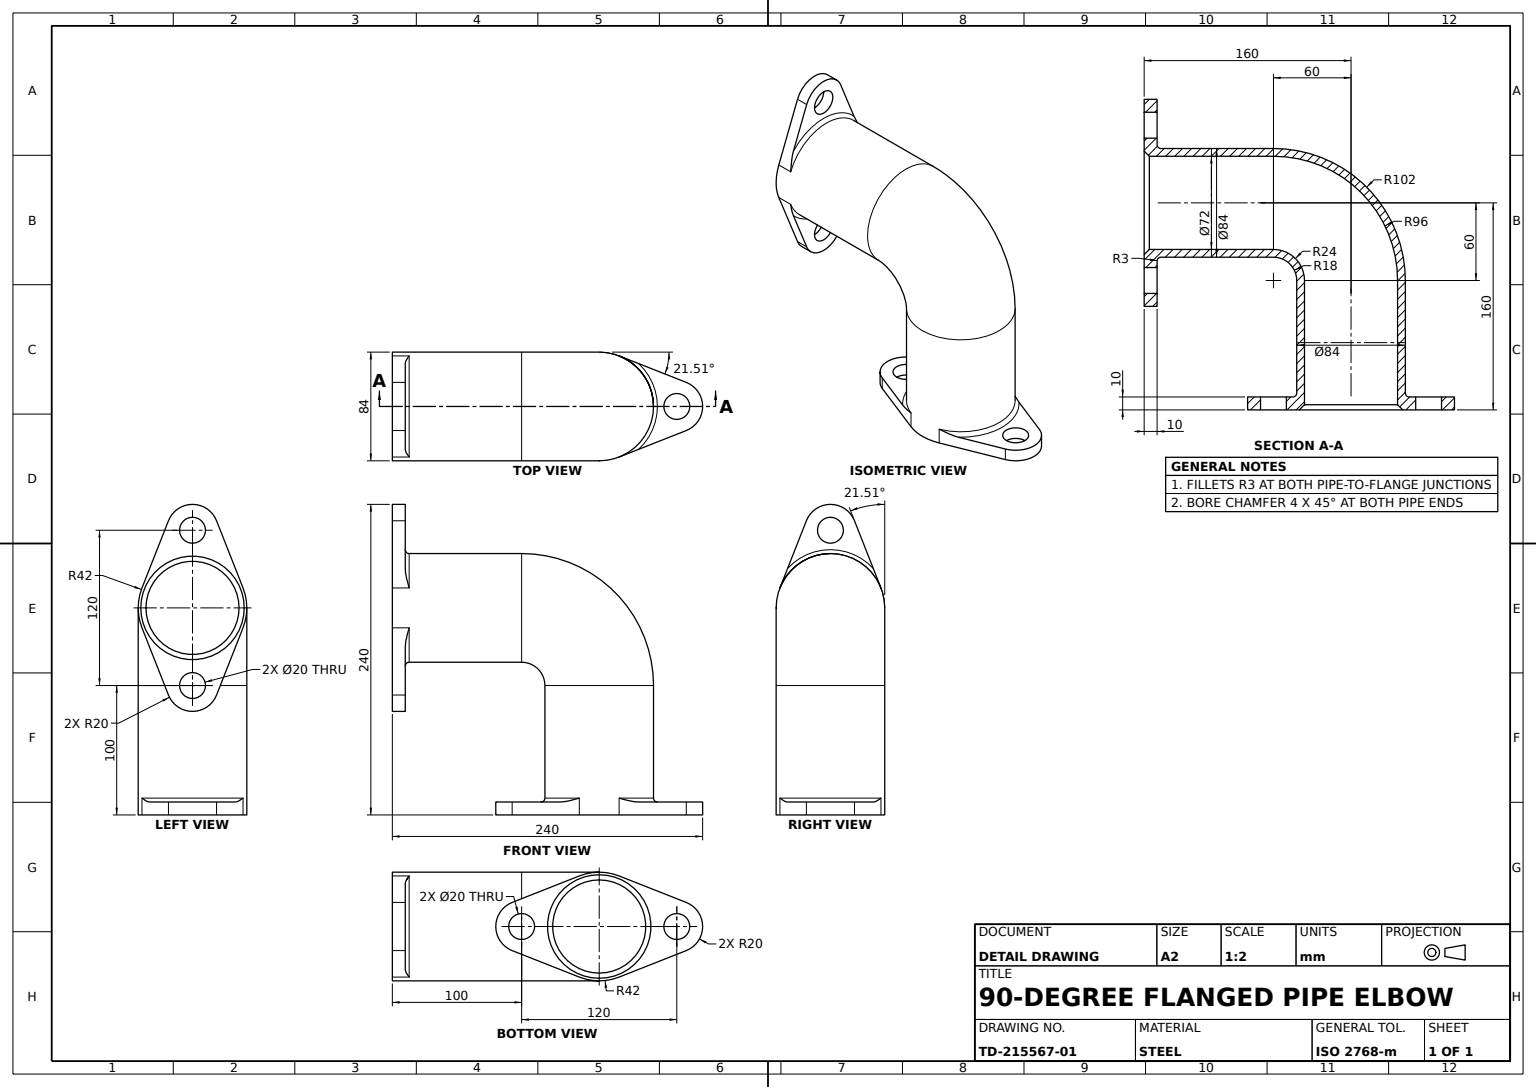
ISO-10303-21;
HEADER;
FILE_DESCRIPTION((''),'2;1');
FILE_NAME('','',(''),(''),'','','');
FILE_SCHEMA(('AUTOMOTIVE_DESIGN'));
ENDSEC;
DATA;
#1=APPLICATION_CONTEXT('');
#2=PRODUCT_CONTEXT('',#1,'mechanical');
#3=PRODUCT('','','',(#2));
#4=PRODUCT_DEFINITION_FORMATION('','',#3);
#5=PRODUCT_DEFINITION_CONTEXT('',#1,'design');
#6=PRODUCT_DEFINITION('','',#4,#5);
#7=PRODUCT_DEFINITION_SHAPE('','',#6);
#8=(LENGTH_UNIT()NAMED_UNIT(*)SI_UNIT(.MILLI.,.METRE.));
#9=(NAMED_UNIT(*)PLANE_ANGLE_UNIT()SI_UNIT($,.RADIAN.));
#10=(NAMED_UNIT(*)SI_UNIT($,.STERADIAN.)SOLID_ANGLE_UNIT());
#11=UNCERTAINTY_MEASURE_WITH_UNIT(LENGTH_MEASURE(1.E-05),#8,'distance_accuracy_value','');
#12=(GEOMETRIC_REPRESENTATION_CONTEXT(3)GLOBAL_UNCERTAINTY_ASSIGNED_CONTEXT((#11))GLOBAL_UNIT_ASSIGNED_CONTEXT((#8,#9,#10))REPRESENTATION_CONTEXT('',''));
#13=CARTESIAN_POINT('',(-150.,110.,0.));
#14=VERTEX_POINT('',#13);
#15=CARTESIAN_POINT('',(-160.,110.,0.));
#16=VERTEX_POINT('',#15);
#17=DIRECTION('',(-1.,0.,0.));
#18=VECTOR('',#17,1000.);
#19=LINE('',#13,#18);
#20=EDGE_CURVE('',#14,#16,#19,.T.);
#21=ORIENTED_EDGE('',*,*,#20,.F.);
#22=CARTESIAN_POINT('',(-150.,90.,0.));
#23=VERTEX_POINT('',#22);
#24=CARTESIAN_POINT('',(-150.,100.,0.));
#25=DIRECTION('',(0.,-1.,0.));
#26=AXIS2_PLACEMENT_3D('',#24,#17,#25);
#27=CIRCLE('',#26,10.);
#28=EDGE_CURVE('',#23,#14,#27,.T.);
#29=ORIENTED_EDGE('',*,*,#28,.F.);
#30=CARTESIAN_POINT('',(-160.,90.,0.));
#31=VERTEX_POINT('',#30);
#32=LINE('',#22,#18);
#33=EDGE_CURVE('',#23,#31,#32,.T.);
#34=ORIENTED_EDGE('',*,*,#33,.T.);
#35=CARTESIAN_POINT('',(-160.,100.,0.));
#36=AXIS2_PLACEMENT_3D('',#35,#17,#25);
#37=CIRCLE('',#36,10.);
#38=EDGE_CURVE('',#31,#16,#37,.T.);
#39=ORIENTED_EDGE('',*,*,#38,.T.);
#40=EDGE_LOOP('',(#21,#29,#34,#39));
#41=FACE_OUTER_BOUND('',#40,.T.);
#42=CYLINDRICAL_SURFACE('',#26,10.);
#43=ADVANCED_FACE('',(#41),#42,.F.);
#44=CARTESIAN_POINT('',(67.333333,10.,-18.607048));
#45=VERTEX_POINT('',#44);
#46=CARTESIAN_POINT('',(67.333333,10.,18.607048));
#47=VERTEX_POINT('',#46);
#48=CARTESIAN_POINT('',(60.,10.,0.));
#49=DIRECTION('',(0.,0.,-1.));
#50=AXIS2_PLACEMENT_3D('',#48,#25,#49);
#51=CIRCLE('',#50,20.);
#52=EDGE_CURVE('',#45,#47,#51,.T.);
#53=ORIENTED_EDGE('',*,*,#52,.T.);
#54=CARTESIAN_POINT('',(67.333333,0.,18.607048));
#55=VERTEX_POINT('',#54);
#56=VECTOR('',#25,1000.);
#57=LINE('',#46,#56);
#58=EDGE_CURVE('',#47,#55,#57,.T.);
#59=ORIENTED_EDGE('',*,*,#58,.T.);
#60=CARTESIAN_POINT('',(67.333333,0.,-18.607048));
#61=VERTEX_POINT('',#60);
#62=CARTESIAN_POINT('',(60.,0.,0.));
#63=AXIS2_PLACEMENT_3D('',#62,#25,#49);
#64=CIRCLE('',#63,20.);
#65=EDGE_CURVE('',#61,#55,#64,.T.);
#66=ORIENTED_EDGE('',*,*,#65,.F.);
#67=LINE('',#44,#56);
#68=EDGE_CURVE('',#45,#61,#67,.T.);
#69=ORIENTED_EDGE('',*,*,#68,.F.);
#70=EDGE_LOOP('',(#53,#59,#66,#69));
#71=FACE_OUTER_BOUND('',#70,.T.);
#72=CYLINDRICAL_SURFACE('',#50,20.);
#73=ADVANCED_FACE('',(#71),#72,.T.);
#74=CARTESIAN_POINT('',(-15.4,13.,-39.0748));
#75=VERTEX_POINT('',#74);
#76=CARTESIAN_POINT('',(-15.4,0.,-39.0748));
#77=VERTEX_POINT('',#76);
#78=CARTESIAN_POINT('',(-15.4,10.,-39.0748));
#79=LINE('',#78,#56);
#80=EDGE_CURVE('',#75,#77,#79,.T.);
#81=ORIENTED_EDGE('',*,*,#80,.T.);
#82=CARTESIAN_POINT('',(-67.333333,0.,-18.607048));
#83=VERTEX_POINT('',#82);
#84=DIRECTION('',(0.930352382,0.,-0.366666667));
#85=VECTOR('',#84,1000.);
#86=LINE('',#82,#85);
#87=EDGE_CURVE('',#83,#77,#86,.T.);
#88=ORIENTED_EDGE('',*,*,#87,.F.);
#89=CARTESIAN_POINT('',(-67.333333,10.,-18.607048));
#90=VERTEX_POINT('',#89);
#91=LINE('',#89,#56);
#92=EDGE_CURVE('',#90,#83,#91,.T.);
#93=ORIENTED_EDGE('',*,*,#92,.F.);
#94=CARTESIAN_POINT('',(-30.430303,10.,-33.151119));
#95=VERTEX_POINT('',#94);
#96=LINE('',#89,#85);
#97=EDGE_CURVE('',#90,#95,#96,.T.);
#98=ORIENTED_EDGE('',*,*,#97,.T.);
#99=CARTESIAN_POINT('',(-29.148292,10.,-33.65638));
#100=CARTESIAN_POINT('',(-27.877079,10.117581,-34.157385));
#101=CARTESIAN_POINT('',(-25.346352,10.480118,-35.154785));
#102=CARTESIAN_POINT('',(-24.08613,10.727695,-35.651458));
#103=CARTESIAN_POINT('',(-21.586323,11.295097,-36.636672));
#104=CARTESIAN_POINT('',(-20.344564,11.61574,-37.126069));
#105=CARTESIAN_POINT('',(-17.86849,12.290793,-38.101929));
#106=CARTESIAN_POINT('',(-16.63255,12.645927,-38.589033));
#107=B_SPLINE_CURVE_WITH_KNOTS('',3,(#94,#99,#100,#101,#102,#103,#104,#105,#106,#74),.UNSPECIFIED.,.F.,.F.,(4,2,2,2,4),(0.,0.004113958,0.008227915,0.012341873,0.016455831),.UNSPECIFIED.);
#108=EDGE_CURVE('',#95,#75,#107,.T.);
#109=ORIENTED_EDGE('',*,*,#108,.T.);
#110=EDGE_LOOP('',(#81,#88,#93,#98,#109));
#111=FACE_OUTER_BOUND('',#110,.T.);
#112=DIRECTION('',(-0.366666667,0.,-0.930352382));
#113=DIRECTION('',(-0.930352382,0.,0.366666667));
#114=AXIS2_PLACEMENT_3D('',#89,#112,#113);
#115=PLANE('',#114);
#116=ADVANCED_FACE('',(#111),#115,.T.);
#117=CARTESIAN_POINT('',(-160.,160.,42.));
#118=VERTEX_POINT('',#117);
#119=CARTESIAN_POINT('',(-160.,175.4,39.0748));
#120=VERTEX_POINT('',#119);
#121=CARTESIAN_POINT('',(-160.,160.,0.));
#122=DIRECTION('',(0.,0.,1.));
#123=AXIS2_PLACEMENT_3D('',#121,#17,#122);
#124=CIRCLE('',#123,42.);
#125=EDGE_CURVE('',#118,#120,#124,.T.);
#126=ORIENTED_EDGE('',*,*,#125,.F.);
#127=CARTESIAN_POINT('',(-60.,160.,42.));
#128=VERTEX_POINT('',#127);
#129=LINE('',#127,#18);
#130=EDGE_CURVE('',#128,#118,#129,.T.);
#131=ORIENTED_EDGE('',*,*,#130,.F.);
#132=CARTESIAN_POINT('',(-60.,202.,0.));
#133=VERTEX_POINT('',#132);
#134=CARTESIAN_POINT('',(-60.,160.,0.));
#135=AXIS2_PLACEMENT_3D('',#134,#17,#122);
#136=CIRCLE('',#135,42.);
#137=EDGE_CURVE('',#128,#133,#136,.T.);
#138=ORIENTED_EDGE('',*,*,#137,.T.);
#139=CARTESIAN_POINT('',(-60.,160.,-42.));
#140=VERTEX_POINT('',#139);
#141=EDGE_CURVE('',#133,#140,#136,.T.);
#142=ORIENTED_EDGE('',*,*,#141,.T.);
#143=CARTESIAN_POINT('',(-160.,160.,-42.));
#144=VERTEX_POINT('',#143);
#145=LINE('',#139,#18);
#146=EDGE_CURVE('',#140,#144,#145,.T.);
#147=ORIENTED_EDGE('',*,*,#146,.T.);
#148=CARTESIAN_POINT('',(-160.,175.4,-39.0748));
#149=VERTEX_POINT('',#148);
#150=EDGE_CURVE('',#149,#144,#124,.T.);
#151=ORIENTED_EDGE('',*,*,#150,.F.);
#152=CARTESIAN_POINT('',(-147.,175.4,-39.0748));
#153=VERTEX_POINT('',#152);
#154=CARTESIAN_POINT('',(-150.,175.4,-39.0748));
#155=LINE('',#154,#18);
#156=EDGE_CURVE('',#153,#149,#155,.T.);
#157=ORIENTED_EDGE('',*,*,#156,.F.);
#158=CARTESIAN_POINT('',(-147.,175.4,39.0748));
#159=VERTEX_POINT('',#158);
#160=CARTESIAN_POINT('',(-147.,160.,0.));
#161=DIRECTION('',(1.,0.,0.));
#162=AXIS2_PLACEMENT_3D('',#160,#161,#25);
#163=CIRCLE('',#162,42.);
#164=EDGE_CURVE('',#153,#159,#163,.T.);
#165=ORIENTED_EDGE('',*,*,#164,.T.);
#166=CARTESIAN_POINT('',(-150.,175.4,39.0748));
#167=LINE('',#166,#18);
#168=EDGE_CURVE('',#159,#120,#167,.T.);
#169=ORIENTED_EDGE('',*,*,#168,.T.);
#170=EDGE_LOOP('',(#126,#131,#138,#142,#147,#151,#157,#165,#169));
#171=FACE_OUTER_BOUND('',#170,.T.);
#172=CYLINDRICAL_SURFACE('',#135,42.);
#173=ADVANCED_FACE('',(#171),#172,.T.);
#174=EDGE_CURVE('',#16,#31,#37,.T.);
#175=ORIENTED_EDGE('',*,*,#174,.T.);
#176=ORIENTED_EDGE('',*,*,#33,.F.);
#177=EDGE_CURVE('',#14,#23,#27,.T.);
#178=ORIENTED_EDGE('',*,*,#177,.F.);
#179=ORIENTED_EDGE('',*,*,#20,.T.);
#180=EDGE_LOOP('',(#175,#176,#178,#179));
#181=FACE_OUTER_BOUND('',#180,.T.);
#182=ADVANCED_FACE('',(#181),#42,.F.);
#183=CARTESIAN_POINT('',(-15.4,13.,39.0748));
#184=VERTEX_POINT('',#183);
#185=CARTESIAN_POINT('',(-15.4,0.,39.0748));
#186=VERTEX_POINT('',#185);
#187=CARTESIAN_POINT('',(-15.4,10.,39.0748));
#188=LINE('',#187,#56);
#189=EDGE_CURVE('',#184,#186,#188,.T.);
#190=ORIENTED_EDGE('',*,*,#189,.F.);
#191=CARTESIAN_POINT('',(-30.430303,10.,33.151119));
#192=VERTEX_POINT('',#191);
#193=CARTESIAN_POINT('',(-17.867552,12.29115,38.102299));
#194=CARTESIAN_POINT('',(-20.336444,11.578792,37.129269));
#195=CARTESIAN_POINT('',(-24.086146,10.727691,35.651452));
#196=CARTESIAN_POINT('',(-25.346364,10.480115,35.15478));
#197=CARTESIAN_POINT('',(-27.877086,10.11758,34.157382));
#198=CARTESIAN_POINT('',(-29.148295,10.,33.656378));
#199=B_SPLINE_CURVE_WITH_KNOTS('',3,(#183,#193,#194,#195,#196,#197,#198,#191),.UNSPECIFIED.,.F.,.F.,(4,2,2,4),(-0.000040988,0.008195114,0.012313165,0.016431215),.UNSPECIFIED.);
#200=EDGE_CURVE('',#184,#192,#199,.T.);
#201=ORIENTED_EDGE('',*,*,#200,.T.);
#202=CARTESIAN_POINT('',(-67.333333,10.,18.607048));
#203=VERTEX_POINT('',#202);
#204=DIRECTION('',(-0.930352382,0.,-0.366666667));
#205=VECTOR('',#204,1000.);
#206=LINE('',#202,#205);
#207=EDGE_CURVE('',#192,#203,#206,.T.);
#208=ORIENTED_EDGE('',*,*,#207,.T.);
#209=CARTESIAN_POINT('',(-67.333333,0.,18.607048));
#210=VERTEX_POINT('',#209);
#211=LINE('',#202,#56);
#212=EDGE_CURVE('',#203,#210,#211,.T.);
#213=ORIENTED_EDGE('',*,*,#212,.T.);
#214=LINE('',#209,#205);
#215=EDGE_CURVE('',#186,#210,#214,.T.);
#216=ORIENTED_EDGE('',*,*,#215,.F.);
#217=EDGE_LOOP('',(#190,#201,#208,#213,#216));
#218=FACE_OUTER_BOUND('',#217,.T.);
#219=DIRECTION('',(-0.366666667,0.,0.930352382));
#220=DIRECTION('',(0.930352382,0.,0.366666667));
#221=AXIS2_PLACEMENT_3D('',#202,#219,#220);
#222=PLANE('',#221);
#223=ADVANCED_FACE('',(#218),#222,.T.);
#224=CARTESIAN_POINT('',(-60.,10.,10.));
#225=VERTEX_POINT('',#224);
#226=CARTESIAN_POINT('',(-60.,10.,-10.));
#227=VERTEX_POINT('',#226);
#228=CARTESIAN_POINT('',(-60.,10.,0.));
#229=AXIS2_PLACEMENT_3D('',#228,#25,#49);
#230=CIRCLE('',#229,10.);
#231=EDGE_CURVE('',#225,#227,#230,.T.);
#232=ORIENTED_EDGE('',*,*,#231,.F.);
#233=CARTESIAN_POINT('',(-60.,0.,10.));
#234=VERTEX_POINT('',#233);
#235=LINE('',#224,#56);
#236=EDGE_CURVE('',#225,#234,#235,.T.);
#237=ORIENTED_EDGE('',*,*,#236,.T.);
#238=CARTESIAN_POINT('',(-60.,0.,-10.));
#239=VERTEX_POINT('',#238);
#240=CARTESIAN_POINT('',(-60.,0.,0.));
#241=AXIS2_PLACEMENT_3D('',#240,#25,#49);
#242=CIRCLE('',#241,10.);
#243=EDGE_CURVE('',#234,#239,#242,.T.);
#244=ORIENTED_EDGE('',*,*,#243,.T.);
#245=LINE('',#226,#56);
#246=EDGE_CURVE('',#227,#239,#245,.T.);
#247=ORIENTED_EDGE('',*,*,#246,.F.);
#248=EDGE_LOOP('',(#232,#237,#244,#247));
#249=FACE_OUTER_BOUND('',#248,.T.);
#250=CYLINDRICAL_SURFACE('',#229,10.);
#251=ADVANCED_FACE('',(#249),#250,.F.);
#252=CARTESIAN_POINT('',(-147.,118.,0.));
#253=VERTEX_POINT('',#252);
#254=CARTESIAN_POINT('',(-147.,144.6,-39.0748));
#255=VERTEX_POINT('',#254);
#256=EDGE_CURVE('',#253,#255,#163,.T.);
#257=ORIENTED_EDGE('',*,*,#256,.F.);
#258=CARTESIAN_POINT('',(-150.,115.,0.));
#259=VERTEX_POINT('',#258);
#260=CARTESIAN_POINT('',(-147.,115.,0.));
#261=AXIS2_PLACEMENT_3D('',#260,#49,#17);
#262=CIRCLE('',#261,3.);
#263=EDGE_CURVE('',#259,#253,#262,.T.);
#264=ORIENTED_EDGE('',*,*,#263,.F.);
#265=CARTESIAN_POINT('',(-150.,129.569697,-33.151119));
#266=VERTEX_POINT('',#265);
#267=CARTESIAN_POINT('',(-150.,160.,0.));
#268=AXIS2_PLACEMENT_3D('',#267,#17,#25);
#269=CIRCLE('',#268,45.);
#270=EDGE_CURVE('',#266,#259,#269,.T.);
#271=ORIENTED_EDGE('',*,*,#270,.F.);
#272=CARTESIAN_POINT('',(-147.70885,142.132448,-38.102299));
#273=CARTESIAN_POINT('',(-148.421208,139.663556,-37.129269));
#274=CARTESIAN_POINT('',(-149.272309,135.913854,-35.651452));
#275=CARTESIAN_POINT('',(-149.519885,134.653636,-35.15478));
#276=CARTESIAN_POINT('',(-149.88242,132.122914,-34.157382));
#277=CARTESIAN_POINT('',(-150.,130.851705,-33.656378));
#278=B_SPLINE_CURVE_WITH_KNOTS('',3,(#254,#272,#273,#274,#275,#276,#277,#265),.UNSPECIFIED.,.F.,.F.,(4,2,2,4),(-0.000040988,0.008195114,0.012313165,0.016431215),.UNSPECIFIED.);
#279=EDGE_CURVE('',#255,#266,#278,.T.);
#280=ORIENTED_EDGE('',*,*,#279,.F.);
#281=EDGE_LOOP('',(#257,#264,#271,#280));
#282=FACE_OUTER_BOUND('',#281,.T.);
#283=AXIS2_PLACEMENT_3D('',#160,#17,#25);
#284=TOROIDAL_SURFACE('',#283,45.,3.);
#285=ADVANCED_FACE('',(#282),#284,.F.);
#286=CARTESIAN_POINT('',(-150.,92.666667,18.607048));
#287=VERTEX_POINT('',#286);
#288=CARTESIAN_POINT('',(-160.,92.666667,18.607048));
#289=VERTEX_POINT('',#288);
#290=LINE('',#286,#18);
#291=EDGE_CURVE('',#287,#289,#290,.T.);
#292=ORIENTED_EDGE('',*,*,#291,.T.);
#293=CARTESIAN_POINT('',(-160.,80.,0.));
#294=VERTEX_POINT('',#293);
#295=CIRCLE('',#36,20.);
#296=EDGE_CURVE('',#294,#289,#295,.T.);
#297=ORIENTED_EDGE('',*,*,#296,.F.);
#298=CARTESIAN_POINT('',(-150.,80.,0.));
#299=VERTEX_POINT('',#298);
#300=LINE('',#298,#18);
#301=EDGE_CURVE('',#299,#294,#300,.T.);
#302=ORIENTED_EDGE('',*,*,#301,.F.);
#303=CIRCLE('',#26,20.);
#304=EDGE_CURVE('',#299,#287,#303,.T.);
#305=ORIENTED_EDGE('',*,*,#304,.T.);
#306=EDGE_LOOP('',(#292,#297,#302,#305));
#307=FACE_OUTER_BOUND('',#306,.T.);
#308=CYLINDRICAL_SURFACE('',#26,20.);
#309=ADVANCED_FACE('',(#307),#308,.T.);
#310=ORIENTED_EDGE('',*,*,#108,.F.);
#311=CARTESIAN_POINT('',(0.,10.,0.));
#312=AXIS2_PLACEMENT_3D('',#311,#25,#49);
#313=CIRCLE('',#312,45.);
#314=EDGE_CURVE('',#192,#95,#313,.T.);
#315=ORIENTED_EDGE('',*,*,#314,.F.);
#316=ORIENTED_EDGE('',*,*,#200,.F.);
#317=CARTESIAN_POINT('',(0.,13.,0.));
#318=DIRECTION('',(0.,1.,0.));
#319=AXIS2_PLACEMENT_3D('',#317,#318,#49);
#320=CIRCLE('',#319,42.);
#321=EDGE_CURVE('',#75,#184,#320,.T.);
#322=ORIENTED_EDGE('',*,*,#321,.F.);
#323=EDGE_LOOP('',(#310,#315,#316,#322));
#324=FACE_OUTER_BOUND('',#323,.T.);
#325=AXIS2_PLACEMENT_3D('',#317,#25,#49);
#326=TOROIDAL_SURFACE('',#325,45.,3.);
#327=ADVANCED_FACE('',(#324),#326,.F.);
#328=CARTESIAN_POINT('',(-150.,92.666667,-18.607048));
#329=VERTEX_POINT('',#328);
#330=CARTESIAN_POINT('',(-150.,144.6,-39.0748));
#331=DIRECTION('',(0.,-0.930352382,0.366666667));
#332=VECTOR('',#331,1000.);
#333=LINE('',#330,#332);
#334=EDGE_CURVE('',#266,#329,#333,.T.);
#335=ORIENTED_EDGE('',*,*,#334,.T.);
#336=CARTESIAN_POINT('',(-160.,92.666667,-18.607048));
#337=VERTEX_POINT('',#336);
#338=LINE('',#328,#18);
#339=EDGE_CURVE('',#329,#337,#338,.T.);
#340=ORIENTED_EDGE('',*,*,#339,.T.);
#341=CARTESIAN_POINT('',(-160.,144.6,-39.0748));
#342=VERTEX_POINT('',#341);
#343=LINE('',#341,#332);
#344=EDGE_CURVE('',#342,#337,#343,.T.);
#345=ORIENTED_EDGE('',*,*,#344,.F.);
#346=LINE('',#330,#18);
#347=EDGE_CURVE('',#255,#342,#346,.T.);
#348=ORIENTED_EDGE('',*,*,#347,.F.);
#349=ORIENTED_EDGE('',*,*,#279,.T.);
#350=EDGE_LOOP('',(#335,#340,#345,#348,#349));
#351=FACE_OUTER_BOUND('',#350,.T.);
#352=DIRECTION('',(0.,-0.366666667,-0.930352382));
#353=DIRECTION('',(0.,0.930352382,-0.366666667));
#354=AXIS2_PLACEMENT_3D('',#330,#352,#353);
#355=PLANE('',#354);
#356=ADVANCED_FACE('',(#351),#355,.T.);
#357=CARTESIAN_POINT('',(-160.,227.333333,-18.607048));
#358=VERTEX_POINT('',#357);
#359=DIRECTION('',(0.,-0.930352382,-0.366666667));
#360=VECTOR('',#359,1000.);
#361=LINE('',#357,#360);
#362=EDGE_CURVE('',#358,#149,#361,.T.);
#363=ORIENTED_EDGE('',*,*,#362,.T.);
#364=ORIENTED_EDGE('',*,*,#150,.T.);
#365=EDGE_CURVE('',#144,#342,#124,.T.);
#366=ORIENTED_EDGE('',*,*,#365,.T.);
#367=ORIENTED_EDGE('',*,*,#344,.T.);
#368=EDGE_CURVE('',#337,#294,#295,.T.);
#369=ORIENTED_EDGE('',*,*,#368,.T.);
#370=ORIENTED_EDGE('',*,*,#296,.T.);
#371=CARTESIAN_POINT('',(-160.,144.6,39.0748));
#372=VERTEX_POINT('',#371);
#373=DIRECTION('',(0.,0.930352382,0.366666667));
#374=VECTOR('',#373,1000.);
#375=LINE('',#288,#374);
#376=EDGE_CURVE('',#289,#372,#375,.T.);
#377=ORIENTED_EDGE('',*,*,#376,.T.);
#378=EDGE_CURVE('',#372,#118,#124,.T.);
#379=ORIENTED_EDGE('',*,*,#378,.T.);
#380=ORIENTED_EDGE('',*,*,#125,.T.);
#381=CARTESIAN_POINT('',(-160.,227.333333,18.607048));
#382=VERTEX_POINT('',#381);
#383=VECTOR('',#353,1000.);
#384=LINE('',#381,#383);
#385=EDGE_CURVE('',#120,#382,#384,.T.);
#386=ORIENTED_EDGE('',*,*,#385,.T.);
#387=CARTESIAN_POINT('',(-160.,220.,0.));
#388=AXIS2_PLACEMENT_3D('',#387,#17,#25);
#389=CIRCLE('',#388,20.);
#390=EDGE_CURVE('',#382,#358,#389,.T.);
#391=ORIENTED_EDGE('',*,*,#390,.T.);
#392=EDGE_LOOP('',(#363,#364,#366,#367,#369,#370,#377,#379,#380,#386,#391));
#393=FACE_OUTER_BOUND('',#392,.T.);
#394=CARTESIAN_POINT('',(-160.,230.,0.));
#395=VERTEX_POINT('',#394);
#396=CARTESIAN_POINT('',(-160.,210.,0.));
#397=VERTEX_POINT('',#396);
#398=CIRCLE('',#388,10.);
#399=EDGE_CURVE('',#395,#397,#398,.T.);
#400=ORIENTED_EDGE('',*,*,#399,.F.);
#401=EDGE_CURVE('',#397,#395,#398,.T.);
#402=ORIENTED_EDGE('',*,*,#401,.F.);
#403=EDGE_LOOP('',(#400,#402));
#404=FACE_BOUND('',#403,.T.);
#405=CARTESIAN_POINT('',(-160.,160.,-40.));
#406=VERTEX_POINT('',#405);
#407=CARTESIAN_POINT('',(-160.,160.,40.));
#408=VERTEX_POINT('',#407);
#409=AXIS2_PLACEMENT_3D('',#121,#161,#122);
#410=CIRCLE('',#409,40.);
#411=EDGE_CURVE('',#406,#408,#410,.T.);
#412=ORIENTED_EDGE('',*,*,#411,.T.);
#413=EDGE_CURVE('',#408,#406,#410,.T.);
#414=ORIENTED_EDGE('',*,*,#413,.T.);
#415=EDGE_LOOP('',(#412,#414));
#416=FACE_BOUND('',#415,.T.);
#417=ORIENTED_EDGE('',*,*,#174,.F.);
#418=ORIENTED_EDGE('',*,*,#38,.F.);
#419=EDGE_LOOP('',(#417,#418));
#420=FACE_BOUND('',#419,.T.);
#421=PLANE('',#123);
#422=ADVANCED_FACE('',(#393,#404,#416,#420),#421,.T.);
#423=CARTESIAN_POINT('',(-150.,129.569697,33.151119));
#424=VERTEX_POINT('',#423);
#425=CARTESIAN_POINT('',(-147.,144.6,39.0748));
#426=VERTEX_POINT('',#425);
#427=CARTESIAN_POINT('',(-150.,130.851708,33.65638));
#428=CARTESIAN_POINT('',(-149.882419,132.122921,34.157385));
#429=CARTESIAN_POINT('',(-149.519882,134.653648,35.154785));
#430=CARTESIAN_POINT('',(-149.272305,135.91387,35.651458));
#431=CARTESIAN_POINT('',(-148.704903,138.413677,36.636672));
#432=CARTESIAN_POINT('',(-148.38426,139.655436,37.126069));
#433=CARTESIAN_POINT('',(-147.709207,142.13151,38.101929));
#434=CARTESIAN_POINT('',(-147.354073,143.36745,38.589033));
#435=B_SPLINE_CURVE_WITH_KNOTS('',3,(#423,#427,#428,#429,#430,#431,#432,#433,#434,#425),.UNSPECIFIED.,.F.,.F.,(4,2,2,2,4),(0.,0.004113958,0.008227915,0.012341873,0.016455831),.UNSPECIFIED.);
#436=EDGE_CURVE('',#424,#426,#435,.T.);
#437=ORIENTED_EDGE('',*,*,#436,.F.);
#438=EDGE_CURVE('',#259,#424,#269,.T.);
#439=ORIENTED_EDGE('',*,*,#438,.F.);
#440=ORIENTED_EDGE('',*,*,#263,.T.);
#441=EDGE_CURVE('',#426,#253,#163,.T.);
#442=ORIENTED_EDGE('',*,*,#441,.F.);
#443=EDGE_LOOP('',(#437,#439,#440,#442));
#444=FACE_OUTER_BOUND('',#443,.T.);
#445=ADVANCED_FACE('',(#444),#284,.F.);
#446=CARTESIAN_POINT('',(0.,4.,-36.));
#447=VERTEX_POINT('',#446);
#448=CARTESIAN_POINT('',(0.,0.,-40.));
#449=VERTEX_POINT('',#448);
#450=DIRECTION('',(0.,-0.707106781,-0.707106781));
#451=VECTOR('',#450,1000.);
#452=LINE('',#448,#451);
#453=EDGE_CURVE('',#447,#449,#452,.T.);
#454=ORIENTED_EDGE('',*,*,#453,.F.);
#455=CARTESIAN_POINT('',(0.,4.,36.));
#456=VERTEX_POINT('',#455);
#457=CARTESIAN_POINT('',(0.,4.,0.));
#458=AXIS2_PLACEMENT_3D('',#457,#25,#122);
#459=CIRCLE('',#458,36.);
#460=EDGE_CURVE('',#456,#447,#459,.T.);
#461=ORIENTED_EDGE('',*,*,#460,.F.);
#462=CARTESIAN_POINT('',(0.,0.,40.));
#463=VERTEX_POINT('',#462);
#464=DIRECTION('',(0.,-0.707106781,0.707106781));
#465=VECTOR('',#464,1000.);
#466=LINE('',#462,#465);
#467=EDGE_CURVE('',#456,#463,#466,.T.);
#468=ORIENTED_EDGE('',*,*,#467,.T.);
#469=CARTESIAN_POINT('',(0.,0.,0.));
#470=AXIS2_PLACEMENT_3D('',#469,#318,#122);
#471=CIRCLE('',#470,40.);
#472=EDGE_CURVE('',#449,#463,#471,.T.);
#473=ORIENTED_EDGE('',*,*,#472,.F.);
#474=EDGE_LOOP('',(#454,#461,#468,#473));
#475=FACE_OUTER_BOUND('',#474,.T.);
#476=AXIS2_PLACEMENT_3D('',#469,#25,#49);
#477=CONICAL_SURFACE('',#476,40.,0.785398163);
#478=ADVANCED_FACE('',(#475),#477,.F.);
#479=ORIENTED_EDGE('',*,*,#401,.T.);
#480=CARTESIAN_POINT('',(-150.,230.,0.));
#481=VERTEX_POINT('',#480);
#482=LINE('',#480,#18);
#483=EDGE_CURVE('',#481,#395,#482,.T.);
#484=ORIENTED_EDGE('',*,*,#483,.F.);
#485=CARTESIAN_POINT('',(-150.,210.,0.));
#486=VERTEX_POINT('',#485);
#487=CARTESIAN_POINT('',(-150.,220.,0.));
#488=AXIS2_PLACEMENT_3D('',#487,#17,#25);
#489=CIRCLE('',#488,10.);
#490=EDGE_CURVE('',#486,#481,#489,.T.);
#491=ORIENTED_EDGE('',*,*,#490,.F.);
#492=LINE('',#485,#18);
#493=EDGE_CURVE('',#486,#397,#492,.T.);
#494=ORIENTED_EDGE('',*,*,#493,.T.);
#495=EDGE_LOOP('',(#479,#484,#491,#494));
#496=FACE_OUTER_BOUND('',#495,.T.);
#497=CYLINDRICAL_SURFACE('',#488,10.);
#498=ADVANCED_FACE('',(#496),#497,.F.);
#499=CARTESIAN_POINT('',(15.4,0.,39.0748));
#500=VERTEX_POINT('',#499);
#501=VECTOR('',#113,1000.);
#502=LINE('',#499,#501);
#503=EDGE_CURVE('',#55,#500,#502,.T.);
#504=ORIENTED_EDGE('',*,*,#503,.T.);
#505=CARTESIAN_POINT('',(0.,0.,42.));
#506=VERTEX_POINT('',#505);
#507=CIRCLE('',#470,42.);
#508=EDGE_CURVE('',#506,#500,#507,.T.);
#509=ORIENTED_EDGE('',*,*,#508,.F.);
#510=EDGE_CURVE('',#186,#506,#507,.T.);
#511=ORIENTED_EDGE('',*,*,#510,.F.);
#512=ORIENTED_EDGE('',*,*,#215,.T.);
#513=CIRCLE('',#241,20.);
#514=EDGE_CURVE('',#210,#83,#513,.T.);
#515=ORIENTED_EDGE('',*,*,#514,.T.);
#516=ORIENTED_EDGE('',*,*,#87,.T.);
#517=CARTESIAN_POINT('',(0.,0.,-42.));
#518=VERTEX_POINT('',#517);
#519=EDGE_CURVE('',#518,#77,#507,.T.);
#520=ORIENTED_EDGE('',*,*,#519,.F.);
#521=CARTESIAN_POINT('',(15.4,0.,-39.0748));
#522=VERTEX_POINT('',#521);
#523=EDGE_CURVE('',#522,#518,#507,.T.);
#524=ORIENTED_EDGE('',*,*,#523,.F.);
#525=VECTOR('',#220,1000.);
#526=LINE('',#521,#525);
#527=EDGE_CURVE('',#522,#61,#526,.T.);
#528=ORIENTED_EDGE('',*,*,#527,.T.);
#529=ORIENTED_EDGE('',*,*,#65,.T.);
#530=EDGE_LOOP('',(#504,#509,#511,#512,#515,#516,#520,#524,#528,#529));
#531=FACE_OUTER_BOUND('',#530,.T.);
#532=EDGE_CURVE('',#463,#449,#471,.T.);
#533=ORIENTED_EDGE('',*,*,#532,.T.);
#534=ORIENTED_EDGE('',*,*,#472,.T.);
#535=EDGE_LOOP('',(#533,#534));
#536=FACE_BOUND('',#535,.T.);
#537=CARTESIAN_POINT('',(60.,0.,10.));
#538=VERTEX_POINT('',#537);
#539=CARTESIAN_POINT('',(60.,0.,-10.));
#540=VERTEX_POINT('',#539);
#541=CIRCLE('',#63,10.);
#542=EDGE_CURVE('',#538,#540,#541,.T.);
#543=ORIENTED_EDGE('',*,*,#542,.F.);
#544=EDGE_CURVE('',#540,#538,#541,.T.);
#545=ORIENTED_EDGE('',*,*,#544,.F.);
#546=EDGE_LOOP('',(#543,#545));
#547=FACE_BOUND('',#546,.T.);
#548=EDGE_CURVE('',#239,#234,#242,.T.);
#549=ORIENTED_EDGE('',*,*,#548,.F.);
#550=ORIENTED_EDGE('',*,*,#243,.F.);
#551=EDGE_LOOP('',(#549,#550));
#552=FACE_BOUND('',#551,.T.);
#553=PLANE('',#470);
#554=ADVANCED_FACE('',(#531,#536,#547,#552),#553,.F.);
#555=CARTESIAN_POINT('',(-150.,227.333333,18.607048));
#556=VERTEX_POINT('',#555);
#557=CARTESIAN_POINT('',(-150.,227.333333,-18.607048));
#558=VERTEX_POINT('',#557);
#559=CIRCLE('',#488,20.);
#560=EDGE_CURVE('',#556,#558,#559,.T.);
#561=ORIENTED_EDGE('',*,*,#560,.T.);
#562=LINE('',#557,#18);
#563=EDGE_CURVE('',#558,#358,#562,.T.);
#564=ORIENTED_EDGE('',*,*,#563,.T.);
#565=ORIENTED_EDGE('',*,*,#390,.F.);
#566=LINE('',#555,#18);
#567=EDGE_CURVE('',#556,#382,#566,.T.);
#568=ORIENTED_EDGE('',*,*,#567,.F.);
#569=EDGE_LOOP('',(#561,#564,#565,#568));
#570=FACE_OUTER_BOUND('',#569,.T.);
#571=CYLINDRICAL_SURFACE('',#488,20.);
#572=ADVANCED_FACE('',(#570),#571,.T.);
#573=ORIENTED_EDGE('',*,*,#231,.T.);
#574=EDGE_CURVE('',#227,#225,#230,.T.);
#575=ORIENTED_EDGE('',*,*,#574,.T.);
#576=EDGE_LOOP('',(#573,#575));
#577=FACE_BOUND('',#576,.T.);
#578=ORIENTED_EDGE('',*,*,#97,.F.);
#579=CIRCLE('',#229,20.);
#580=EDGE_CURVE('',#203,#90,#579,.T.);
#581=ORIENTED_EDGE('',*,*,#580,.F.);
#582=ORIENTED_EDGE('',*,*,#207,.F.);
#583=ORIENTED_EDGE('',*,*,#314,.T.);
#584=EDGE_LOOP('',(#578,#581,#582,#583));
#585=FACE_OUTER_BOUND('',#584,.T.);
#586=PLANE('',#312);
#587=ADVANCED_FACE('',(#577,#585),#586,.F.);
#588=ORIENTED_EDGE('',*,*,#544,.T.);
#589=CARTESIAN_POINT('',(60.,10.,10.));
#590=VERTEX_POINT('',#589);
#591=LINE('',#589,#56);
#592=EDGE_CURVE('',#590,#538,#591,.T.);
#593=ORIENTED_EDGE('',*,*,#592,.F.);
#594=CARTESIAN_POINT('',(60.,10.,-10.));
#595=VERTEX_POINT('',#594);
#596=CIRCLE('',#50,10.);
#597=EDGE_CURVE('',#595,#590,#596,.T.);
#598=ORIENTED_EDGE('',*,*,#597,.F.);
#599=LINE('',#594,#56);
#600=EDGE_CURVE('',#595,#540,#599,.T.);
#601=ORIENTED_EDGE('',*,*,#600,.T.);
#602=EDGE_LOOP('',(#588,#593,#598,#601));
#603=FACE_OUTER_BOUND('',#602,.T.);
#604=CYLINDRICAL_SURFACE('',#50,10.);
#605=ADVANCED_FACE('',(#603),#604,.F.);
#606=CARTESIAN_POINT('',(15.4,13.,-39.0748));
#607=VERTEX_POINT('',#606);
#608=CARTESIAN_POINT('',(15.4,10.,-39.0748));
#609=LINE('',#608,#56);
#610=EDGE_CURVE('',#607,#522,#609,.T.);
#611=ORIENTED_EDGE('',*,*,#610,.F.);
#612=CARTESIAN_POINT('',(30.430303,10.,-33.151119));
#613=VERTEX_POINT('',#612);
#614=CARTESIAN_POINT('',(17.867552,12.29115,-38.102299));
#615=CARTESIAN_POINT('',(20.336444,11.578792,-37.129269));
#616=CARTESIAN_POINT('',(24.086146,10.727691,-35.651452));
#617=CARTESIAN_POINT('',(25.346364,10.480115,-35.15478));
#618=CARTESIAN_POINT('',(27.877086,10.11758,-34.157382));
#619=CARTESIAN_POINT('',(29.148295,10.,-33.656378));
#620=B_SPLINE_CURVE_WITH_KNOTS('',3,(#606,#614,#615,#616,#617,#618,#619,#612),.UNSPECIFIED.,.F.,.F.,(4,2,2,4),(-0.000040988,0.008195114,0.012313165,0.016431215),.UNSPECIFIED.);
#621=EDGE_CURVE('',#607,#613,#620,.T.);
#622=ORIENTED_EDGE('',*,*,#621,.T.);
#623=LINE('',#608,#525);
#624=EDGE_CURVE('',#613,#45,#623,.T.);
#625=ORIENTED_EDGE('',*,*,#624,.T.);
#626=ORIENTED_EDGE('',*,*,#68,.T.);
#627=ORIENTED_EDGE('',*,*,#527,.F.);
#628=EDGE_LOOP('',(#611,#622,#625,#626,#627));
#629=FACE_OUTER_BOUND('',#628,.T.);
#630=DIRECTION('',(0.366666667,0.,-0.930352382));
#631=AXIS2_PLACEMENT_3D('',#608,#630,#204);
#632=PLANE('',#631);
#633=ADVANCED_FACE('',(#629),#632,.T.);
#634=CARTESIAN_POINT('',(15.4,13.,39.0748));
#635=VERTEX_POINT('',#634);
#636=CARTESIAN_POINT('',(15.4,10.,39.0748));
#637=LINE('',#636,#56);
#638=EDGE_CURVE('',#635,#500,#637,.T.);
#639=ORIENTED_EDGE('',*,*,#638,.T.);
#640=ORIENTED_EDGE('',*,*,#503,.F.);
#641=ORIENTED_EDGE('',*,*,#58,.F.);
#642=CARTESIAN_POINT('',(30.430303,10.,33.151119));
#643=VERTEX_POINT('',#642);
#644=LINE('',#636,#501);
#645=EDGE_CURVE('',#47,#643,#644,.T.);
#646=ORIENTED_EDGE('',*,*,#645,.T.);
#647=CARTESIAN_POINT('',(29.148292,10.,33.65638));
#648=CARTESIAN_POINT('',(27.877079,10.117581,34.157385));
#649=CARTESIAN_POINT('',(25.346352,10.480118,35.154785));
#650=CARTESIAN_POINT('',(24.08613,10.727695,35.651458));
#651=CARTESIAN_POINT('',(21.586323,11.295097,36.636672));
#652=CARTESIAN_POINT('',(20.344564,11.61574,37.126069));
#653=CARTESIAN_POINT('',(17.86849,12.290793,38.101929));
#654=CARTESIAN_POINT('',(16.63255,12.645927,38.589033));
#655=B_SPLINE_CURVE_WITH_KNOTS('',3,(#642,#647,#648,#649,#650,#651,#652,#653,#654,#634),.UNSPECIFIED.,.F.,.F.,(4,2,2,2,4),(0.,0.004113958,0.008227915,0.012341873,0.016455831),.UNSPECIFIED.);
#656=EDGE_CURVE('',#643,#635,#655,.T.);
#657=ORIENTED_EDGE('',*,*,#656,.T.);
#658=EDGE_LOOP('',(#639,#640,#641,#646,#657));
#659=FACE_OUTER_BOUND('',#658,.T.);
#660=DIRECTION('',(0.366666667,0.,0.930352382));
#661=AXIS2_PLACEMENT_3D('',#636,#660,#84);
#662=PLANE('',#661);
#663=ADVANCED_FACE('',(#659),#662,.T.);
#664=ORIENTED_EDGE('',*,*,#460,.T.);
#665=CARTESIAN_POINT('',(0.,100.,-36.));
#666=VERTEX_POINT('',#665);
#667=CARTESIAN_POINT('',(0.,0.,-36.));
#668=VECTOR('',#318,1000.);
#669=LINE('',#667,#668);
#670=EDGE_CURVE('',#447,#666,#669,.T.);
#671=ORIENTED_EDGE('',*,*,#670,.T.);
#672=CARTESIAN_POINT('',(-36.,100.,0.));
#673=VERTEX_POINT('',#672);
#674=CARTESIAN_POINT('',(0.,100.,0.));
#675=AXIS2_PLACEMENT_3D('',#674,#318,#122);
#676=CIRCLE('',#675,36.);
#677=EDGE_CURVE('',#666,#673,#676,.T.);
#678=ORIENTED_EDGE('',*,*,#677,.T.);
#679=CARTESIAN_POINT('',(0.,100.,36.));
#680=VERTEX_POINT('',#679);
#681=EDGE_CURVE('',#673,#680,#676,.T.);
#682=ORIENTED_EDGE('',*,*,#681,.T.);
#683=CARTESIAN_POINT('',(0.,0.,36.));
#684=LINE('',#683,#668);
#685=EDGE_CURVE('',#456,#680,#684,.T.);
#686=ORIENTED_EDGE('',*,*,#685,.F.);
#687=EDGE_LOOP('',(#664,#671,#678,#682,#686));
#688=FACE_OUTER_BOUND('',#687,.T.);
#689=CYLINDRICAL_SURFACE('',#470,36.);
#690=ADVANCED_FACE('',(#688),#689,.F.);
#691=CARTESIAN_POINT('',(-156.,160.,36.));
#692=VERTEX_POINT('',#691);
#693=CARTESIAN_POINT('',(-156.,160.,-36.));
#694=VERTEX_POINT('',#693);
#695=CARTESIAN_POINT('',(-156.,160.,0.));
#696=AXIS2_PLACEMENT_3D('',#695,#17,#122);
#697=CIRCLE('',#696,36.);
#698=EDGE_CURVE('',#692,#694,#697,.T.);
#699=ORIENTED_EDGE('',*,*,#698,.T.);
#700=CARTESIAN_POINT('',(-60.,160.,-36.));
#701=VERTEX_POINT('',#700);
#702=LINE('',#700,#18);
#703=EDGE_CURVE('',#701,#694,#702,.T.);
#704=ORIENTED_EDGE('',*,*,#703,.F.);
#705=CARTESIAN_POINT('',(-60.,196.,0.));
#706=VERTEX_POINT('',#705);
#707=CIRCLE('',#135,36.);
#708=EDGE_CURVE('',#706,#701,#707,.T.);
#709=ORIENTED_EDGE('',*,*,#708,.F.);
#710=CARTESIAN_POINT('',(-60.,160.,36.));
#711=VERTEX_POINT('',#710);
#712=EDGE_CURVE('',#711,#706,#707,.T.);
#713=ORIENTED_EDGE('',*,*,#712,.F.);
#714=LINE('',#710,#18);
#715=EDGE_CURVE('',#711,#692,#714,.T.);
#716=ORIENTED_EDGE('',*,*,#715,.T.);
#717=EDGE_LOOP('',(#699,#704,#709,#713,#716));
#718=FACE_OUTER_BOUND('',#717,.T.);
#719=CYLINDRICAL_SURFACE('',#135,36.);
#720=ADVANCED_FACE('',(#718),#719,.F.);
#721=ORIENTED_EDGE('',*,*,#574,.F.);
#722=ORIENTED_EDGE('',*,*,#246,.T.);
#723=ORIENTED_EDGE('',*,*,#548,.T.);
#724=ORIENTED_EDGE('',*,*,#236,.F.);
#725=EDGE_LOOP('',(#721,#722,#723,#724));
#726=FACE_OUTER_BOUND('',#725,.T.);
#727=ADVANCED_FACE('',(#726),#250,.F.);
#728=ORIENTED_EDGE('',*,*,#600,.F.);
#729=EDGE_CURVE('',#590,#595,#596,.T.);
#730=ORIENTED_EDGE('',*,*,#729,.F.);
#731=ORIENTED_EDGE('',*,*,#592,.T.);
#732=ORIENTED_EDGE('',*,*,#542,.T.);
#733=EDGE_LOOP('',(#728,#730,#731,#732));
#734=FACE_OUTER_BOUND('',#733,.T.);
#735=ADVANCED_FACE('',(#734),#604,.F.);
#736=CARTESIAN_POINT('',(36.,100.,0.));
#737=VERTEX_POINT('',#736);
#738=EDGE_CURVE('',#680,#737,#676,.T.);
#739=ORIENTED_EDGE('',*,*,#738,.T.);
#740=EDGE_CURVE('',#737,#666,#676,.T.);
#741=ORIENTED_EDGE('',*,*,#740,.T.);
#742=ORIENTED_EDGE('',*,*,#670,.F.);
#743=EDGE_CURVE('',#447,#456,#459,.T.);
#744=ORIENTED_EDGE('',*,*,#743,.T.);
#745=ORIENTED_EDGE('',*,*,#685,.T.);
#746=EDGE_LOOP('',(#739,#741,#742,#744,#745));
#747=FACE_OUTER_BOUND('',#746,.T.);
#748=ADVANCED_FACE('',(#747),#689,.F.);
#749=EDGE_CURVE('',#613,#643,#313,.T.);
#750=ORIENTED_EDGE('',*,*,#749,.T.);
#751=ORIENTED_EDGE('',*,*,#645,.F.);
#752=ORIENTED_EDGE('',*,*,#52,.F.);
#753=ORIENTED_EDGE('',*,*,#624,.F.);
#754=EDGE_LOOP('',(#750,#751,#752,#753));
#755=FACE_OUTER_BOUND('',#754,.T.);
#756=ORIENTED_EDGE('',*,*,#729,.T.);
#757=ORIENTED_EDGE('',*,*,#597,.T.);
#758=EDGE_LOOP('',(#756,#757));
#759=FACE_BOUND('',#758,.T.);
#760=ADVANCED_FACE('',(#755,#759),#586,.F.);
#761=ORIENTED_EDGE('',*,*,#677,.F.);
#762=ORIENTED_EDGE('',*,*,#740,.F.);
#763=CARTESIAN_POINT('',(-60.,100.,0.));
#764=AXIS2_PLACEMENT_3D('',#763,#122,#161);
#765=CIRCLE('',#764,96.);
#766=EDGE_CURVE('',#737,#706,#765,.T.);
#767=ORIENTED_EDGE('',*,*,#766,.T.);
#768=ORIENTED_EDGE('',*,*,#708,.T.);
#769=CARTESIAN_POINT('',(-60.,124.,0.));
#770=VERTEX_POINT('',#769);
#771=EDGE_CURVE('',#701,#770,#707,.T.);
#772=ORIENTED_EDGE('',*,*,#771,.T.);
#773=CIRCLE('',#764,24.);
#774=EDGE_CURVE('',#673,#770,#773,.T.);
#775=ORIENTED_EDGE('',*,*,#774,.F.);
#776=EDGE_LOOP('',(#761,#762,#767,#768,#772,#775));
#777=FACE_OUTER_BOUND('',#776,.T.);
#778=TOROIDAL_SURFACE('',#764,60.,36.);
#779=ADVANCED_FACE('',(#777),#778,.F.);
#780=ORIENTED_EDGE('',*,*,#712,.T.);
#781=ORIENTED_EDGE('',*,*,#766,.F.);
#782=ORIENTED_EDGE('',*,*,#738,.F.);
#783=ORIENTED_EDGE('',*,*,#681,.F.);
#784=ORIENTED_EDGE('',*,*,#774,.T.);
#785=EDGE_CURVE('',#770,#711,#707,.T.);
#786=ORIENTED_EDGE('',*,*,#785,.T.);
#787=EDGE_LOOP('',(#780,#781,#782,#783,#784,#786));
#788=FACE_OUTER_BOUND('',#787,.T.);
#789=ADVANCED_FACE('',(#788),#778,.F.);
#790=ORIENTED_EDGE('',*,*,#368,.F.);
#791=ORIENTED_EDGE('',*,*,#339,.F.);
#792=EDGE_CURVE('',#329,#299,#303,.T.);
#793=ORIENTED_EDGE('',*,*,#792,.T.);
#794=ORIENTED_EDGE('',*,*,#301,.T.);
#795=EDGE_LOOP('',(#790,#791,#793,#794));
#796=FACE_OUTER_BOUND('',#795,.T.);
#797=ADVANCED_FACE('',(#796),#308,.T.);
#798=DIRECTION('',(-0.707106781,0.,-0.707106781));
#799=VECTOR('',#798,1000.);
#800=LINE('',#693,#799);
#801=EDGE_CURVE('',#694,#406,#800,.T.);
#802=ORIENTED_EDGE('',*,*,#801,.F.);
#803=ORIENTED_EDGE('',*,*,#698,.F.);
#804=DIRECTION('',(-0.707106781,0.,0.707106781));
#805=VECTOR('',#804,1000.);
#806=LINE('',#691,#805);
#807=EDGE_CURVE('',#692,#408,#806,.T.);
#808=ORIENTED_EDGE('',*,*,#807,.T.);
#809=ORIENTED_EDGE('',*,*,#411,.F.);
#810=EDGE_LOOP('',(#802,#803,#808,#809));
#811=FACE_OUTER_BOUND('',#810,.T.);
#812=CONICAL_SURFACE('',#696,36.,0.785398163);
#813=ADVANCED_FACE('',(#811),#812,.F.);
#814=EDGE_CURVE('',#481,#486,#489,.T.);
#815=ORIENTED_EDGE('',*,*,#814,.F.);
#816=ORIENTED_EDGE('',*,*,#483,.T.);
#817=ORIENTED_EDGE('',*,*,#399,.T.);
#818=ORIENTED_EDGE('',*,*,#493,.F.);
#819=EDGE_LOOP('',(#815,#816,#817,#818));
#820=FACE_OUTER_BOUND('',#819,.T.);
#821=ADVANCED_FACE('',(#820),#497,.F.);
#822=ORIENTED_EDGE('',*,*,#141,.F.);
#823=CARTESIAN_POINT('',(42.,100.,0.));
#824=VERTEX_POINT('',#823);
#825=CIRCLE('',#764,102.);
#826=EDGE_CURVE('',#824,#133,#825,.T.);
#827=ORIENTED_EDGE('',*,*,#826,.F.);
#828=CARTESIAN_POINT('',(0.,100.,-42.));
#829=VERTEX_POINT('',#828);
#830=AXIS2_PLACEMENT_3D('',#674,#318,#49);
#831=CIRCLE('',#830,42.);
#832=EDGE_CURVE('',#824,#829,#831,.T.);
#833=ORIENTED_EDGE('',*,*,#832,.T.);
#834=CARTESIAN_POINT('',(-42.,100.,0.));
#835=VERTEX_POINT('',#834);
#836=EDGE_CURVE('',#829,#835,#831,.T.);
#837=ORIENTED_EDGE('',*,*,#836,.T.);
#838=CARTESIAN_POINT('',(-60.,118.,0.));
#839=VERTEX_POINT('',#838);
#840=CIRCLE('',#764,18.);
#841=EDGE_CURVE('',#835,#839,#840,.T.);
#842=ORIENTED_EDGE('',*,*,#841,.T.);
#843=EDGE_CURVE('',#140,#839,#136,.T.);
#844=ORIENTED_EDGE('',*,*,#843,.F.);
#845=EDGE_LOOP('',(#822,#827,#833,#837,#842,#844));
#846=FACE_OUTER_BOUND('',#845,.T.);
#847=TOROIDAL_SURFACE('',#764,60.,42.);
#848=ADVANCED_FACE('',(#846),#847,.T.);
#849=ORIENTED_EDGE('',*,*,#168,.F.);
#850=CARTESIAN_POINT('',(-150.,190.430303,33.151119));
#851=VERTEX_POINT('',#850);
#852=CARTESIAN_POINT('',(-147.70885,177.867552,38.102299));
#853=CARTESIAN_POINT('',(-148.421208,180.336444,37.129269));
#854=CARTESIAN_POINT('',(-149.272309,184.086146,35.651452));
#855=CARTESIAN_POINT('',(-149.519885,185.346364,35.15478));
#856=CARTESIAN_POINT('',(-149.88242,187.877086,34.157382));
#857=CARTESIAN_POINT('',(-150.,189.148295,33.656378));
#858=B_SPLINE_CURVE_WITH_KNOTS('',3,(#158,#852,#853,#854,#855,#856,#857,#850),.UNSPECIFIED.,.F.,.F.,(4,2,2,4),(-0.000040988,0.008195114,0.012313165,0.016431215),.UNSPECIFIED.);
#859=EDGE_CURVE('',#159,#851,#858,.T.);
#860=ORIENTED_EDGE('',*,*,#859,.T.);
#861=LINE('',#555,#383);
#862=EDGE_CURVE('',#851,#556,#861,.T.);
#863=ORIENTED_EDGE('',*,*,#862,.T.);
#864=ORIENTED_EDGE('',*,*,#567,.T.);
#865=ORIENTED_EDGE('',*,*,#385,.F.);
#866=EDGE_LOOP('',(#849,#860,#863,#864,#865));
#867=FACE_OUTER_BOUND('',#866,.T.);
#868=DIRECTION('',(0.,0.366666667,0.930352382));
#869=AXIS2_PLACEMENT_3D('',#555,#868,#331);
#870=PLANE('',#869);
#871=ADVANCED_FACE('',(#867),#870,.T.);
#872=ORIENTED_EDGE('',*,*,#291,.F.);
#873=LINE('',#286,#374);
#874=EDGE_CURVE('',#287,#424,#873,.T.);
#875=ORIENTED_EDGE('',*,*,#874,.T.);
#876=ORIENTED_EDGE('',*,*,#436,.T.);
#877=CARTESIAN_POINT('',(-150.,144.6,39.0748));
#878=LINE('',#877,#18);
#879=EDGE_CURVE('',#426,#372,#878,.T.);
#880=ORIENTED_EDGE('',*,*,#879,.T.);
#881=ORIENTED_EDGE('',*,*,#376,.F.);
#882=EDGE_LOOP('',(#872,#875,#876,#880,#881));
#883=FACE_OUTER_BOUND('',#882,.T.);
#884=DIRECTION('',(0.,-0.366666667,0.930352382));
#885=AXIS2_PLACEMENT_3D('',#286,#884,#359);
#886=PLANE('',#885);
#887=ADVANCED_FACE('',(#883),#886,.T.);
#888=ORIENTED_EDGE('',*,*,#832,.F.);
#889=CARTESIAN_POINT('',(0.,100.,42.));
#890=VERTEX_POINT('',#889);
#891=EDGE_CURVE('',#890,#824,#831,.T.);
#892=ORIENTED_EDGE('',*,*,#891,.F.);
#893=LINE('',#505,#668);
#894=EDGE_CURVE('',#506,#890,#893,.T.);
#895=ORIENTED_EDGE('',*,*,#894,.F.);
#896=ORIENTED_EDGE('',*,*,#508,.T.);
#897=ORIENTED_EDGE('',*,*,#638,.F.);
#898=EDGE_CURVE('',#635,#607,#320,.T.);
#899=ORIENTED_EDGE('',*,*,#898,.T.);
#900=ORIENTED_EDGE('',*,*,#610,.T.);
#901=ORIENTED_EDGE('',*,*,#523,.T.);
#902=LINE('',#517,#668);
#903=EDGE_CURVE('',#518,#829,#902,.T.);
#904=ORIENTED_EDGE('',*,*,#903,.T.);
#905=EDGE_LOOP('',(#888,#892,#895,#896,#897,#899,#900,#901,#904));
#906=FACE_OUTER_BOUND('',#905,.T.);
#907=CYLINDRICAL_SURFACE('',#470,42.);
#908=ADVANCED_FACE('',(#906),#907,.T.);
#909=ORIENTED_EDGE('',*,*,#467,.F.);
#910=ORIENTED_EDGE('',*,*,#743,.F.);
#911=ORIENTED_EDGE('',*,*,#453,.T.);
#912=ORIENTED_EDGE('',*,*,#532,.F.);
#913=EDGE_LOOP('',(#909,#910,#911,#912));
#914=FACE_OUTER_BOUND('',#913,.T.);
#915=ADVANCED_FACE('',(#914),#477,.F.);
#916=ORIENTED_EDGE('',*,*,#560,.F.);
#917=ORIENTED_EDGE('',*,*,#862,.F.);
#918=CARTESIAN_POINT('',(-150.,190.430303,-33.151119));
#919=VERTEX_POINT('',#918);
#920=EDGE_CURVE('',#851,#919,#269,.T.);
#921=ORIENTED_EDGE('',*,*,#920,.T.);
#922=LINE('',#557,#360);
#923=EDGE_CURVE('',#558,#919,#922,.T.);
#924=ORIENTED_EDGE('',*,*,#923,.F.);
#925=EDGE_LOOP('',(#916,#917,#921,#924));
#926=FACE_OUTER_BOUND('',#925,.T.);
#927=ORIENTED_EDGE('',*,*,#814,.T.);
#928=ORIENTED_EDGE('',*,*,#490,.T.);
#929=EDGE_LOOP('',(#927,#928));
#930=FACE_BOUND('',#929,.T.);
#931=PLANE('',#488);
#932=ADVANCED_FACE('',(#926,#930),#931,.F.);
#933=ORIENTED_EDGE('',*,*,#28,.T.);
#934=ORIENTED_EDGE('',*,*,#177,.T.);
#935=EDGE_LOOP('',(#933,#934));
#936=FACE_BOUND('',#935,.T.);
#937=ORIENTED_EDGE('',*,*,#792,.F.);
#938=ORIENTED_EDGE('',*,*,#334,.F.);
#939=ORIENTED_EDGE('',*,*,#270,.T.);
#940=ORIENTED_EDGE('',*,*,#438,.T.);
#941=ORIENTED_EDGE('',*,*,#874,.F.);
#942=ORIENTED_EDGE('',*,*,#304,.F.);
#943=EDGE_LOOP('',(#937,#938,#939,#940,#941,#942));
#944=FACE_OUTER_BOUND('',#943,.T.);
#945=ADVANCED_FACE('',(#936,#944),#931,.F.);
#946=ORIENTED_EDGE('',*,*,#807,.F.);
#947=EDGE_CURVE('',#694,#692,#697,.T.);
#948=ORIENTED_EDGE('',*,*,#947,.F.);
#949=ORIENTED_EDGE('',*,*,#801,.T.);
#950=ORIENTED_EDGE('',*,*,#413,.F.);
#951=EDGE_LOOP('',(#946,#948,#949,#950));
#952=FACE_OUTER_BOUND('',#951,.T.);
#953=ADVANCED_FACE('',(#952),#812,.F.);
#954=ORIENTED_EDGE('',*,*,#947,.T.);
#955=ORIENTED_EDGE('',*,*,#715,.F.);
#956=ORIENTED_EDGE('',*,*,#785,.F.);
#957=ORIENTED_EDGE('',*,*,#771,.F.);
#958=ORIENTED_EDGE('',*,*,#703,.T.);
#959=EDGE_LOOP('',(#954,#955,#956,#957,#958));
#960=FACE_OUTER_BOUND('',#959,.T.);
#961=ADVANCED_FACE('',(#960),#719,.F.);
#962=EDGE_CURVE('',#839,#128,#136,.T.);
#963=ORIENTED_EDGE('',*,*,#962,.T.);
#964=ORIENTED_EDGE('',*,*,#130,.T.);
#965=ORIENTED_EDGE('',*,*,#378,.F.);
#966=ORIENTED_EDGE('',*,*,#879,.F.);
#967=ORIENTED_EDGE('',*,*,#441,.T.);
#968=ORIENTED_EDGE('',*,*,#256,.T.);
#969=ORIENTED_EDGE('',*,*,#347,.T.);
#970=ORIENTED_EDGE('',*,*,#365,.F.);
#971=ORIENTED_EDGE('',*,*,#146,.F.);
#972=ORIENTED_EDGE('',*,*,#843,.T.);
#973=EDGE_LOOP('',(#963,#964,#965,#966,#967,#968,#969,#970,#971,#972));
#974=FACE_OUTER_BOUND('',#973,.T.);
#975=ADVANCED_FACE('',(#974),#172,.T.);
#976=ORIENTED_EDGE('',*,*,#898,.F.);
#977=ORIENTED_EDGE('',*,*,#656,.F.);
#978=ORIENTED_EDGE('',*,*,#749,.F.);
#979=ORIENTED_EDGE('',*,*,#621,.F.);
#980=EDGE_LOOP('',(#976,#977,#978,#979));
#981=FACE_OUTER_BOUND('',#980,.T.);
#982=ADVANCED_FACE('',(#981),#326,.F.);
#983=ORIENTED_EDGE('',*,*,#212,.F.);
#984=ORIENTED_EDGE('',*,*,#580,.T.);
#985=ORIENTED_EDGE('',*,*,#92,.T.);
#986=ORIENTED_EDGE('',*,*,#514,.F.);
#987=EDGE_LOOP('',(#983,#984,#985,#986));
#988=FACE_OUTER_BOUND('',#987,.T.);
#989=CYLINDRICAL_SURFACE('',#229,20.);
#990=ADVANCED_FACE('',(#988),#989,.T.);
#991=CARTESIAN_POINT('',(-150.,189.148292,-33.65638));
#992=CARTESIAN_POINT('',(-149.882419,187.877079,-34.157385));
#993=CARTESIAN_POINT('',(-149.519882,185.346352,-35.154785));
#994=CARTESIAN_POINT('',(-149.272305,184.08613,-35.651458));
#995=CARTESIAN_POINT('',(-148.704903,181.586323,-36.636672));
#996=CARTESIAN_POINT('',(-148.38426,180.344564,-37.126069));
#997=CARTESIAN_POINT('',(-147.709207,177.86849,-38.101929));
#998=CARTESIAN_POINT('',(-147.354073,176.63255,-38.589033));
#999=B_SPLINE_CURVE_WITH_KNOTS('',3,(#918,#991,#992,#993,#994,#995,#996,#997,#998,#152),.UNSPECIFIED.,.F.,.F.,(4,2,2,2,4),(0.,0.004113958,0.008227915,0.012341873,0.016455831),.UNSPECIFIED.);
#1000=EDGE_CURVE('',#919,#153,#999,.T.);
#1001=ORIENTED_EDGE('',*,*,#1000,.T.);
#1002=ORIENTED_EDGE('',*,*,#156,.T.);
#1003=ORIENTED_EDGE('',*,*,#362,.F.);
#1004=ORIENTED_EDGE('',*,*,#563,.F.);
#1005=ORIENTED_EDGE('',*,*,#923,.T.);
#1006=EDGE_LOOP('',(#1001,#1002,#1003,#1004,#1005));
#1007=FACE_OUTER_BOUND('',#1006,.T.);
#1008=DIRECTION('',(0.,0.366666667,-0.930352382));
#1009=AXIS2_PLACEMENT_3D('',#557,#1008,#373);
#1010=PLANE('',#1009);
#1011=ADVANCED_FACE('',(#1007),#1010,.T.);
#1012=ORIENTED_EDGE('',*,*,#189,.T.);
#1013=ORIENTED_EDGE('',*,*,#510,.T.);
#1014=ORIENTED_EDGE('',*,*,#894,.T.);
#1015=EDGE_CURVE('',#835,#890,#831,.T.);
#1016=ORIENTED_EDGE('',*,*,#1015,.F.);
#1017=ORIENTED_EDGE('',*,*,#836,.F.);
#1018=ORIENTED_EDGE('',*,*,#903,.F.);
#1019=ORIENTED_EDGE('',*,*,#519,.T.);
#1020=ORIENTED_EDGE('',*,*,#80,.F.);
#1021=ORIENTED_EDGE('',*,*,#321,.T.);
#1022=EDGE_LOOP('',(#1012,#1013,#1014,#1016,#1017,#1018,#1019,#1020,#1021));
#1023=FACE_OUTER_BOUND('',#1022,.T.);
#1024=ADVANCED_FACE('',(#1023),#907,.T.);
#1025=ORIENTED_EDGE('',*,*,#962,.F.);
#1026=ORIENTED_EDGE('',*,*,#841,.F.);
#1027=ORIENTED_EDGE('',*,*,#1015,.T.);
#1028=ORIENTED_EDGE('',*,*,#891,.T.);
#1029=ORIENTED_EDGE('',*,*,#826,.T.);
#1030=ORIENTED_EDGE('',*,*,#137,.F.);
#1031=EDGE_LOOP('',(#1025,#1026,#1027,#1028,#1029,#1030));
#1032=FACE_OUTER_BOUND('',#1031,.T.);
#1033=ADVANCED_FACE('',(#1032),#847,.T.);
#1034=ORIENTED_EDGE('',*,*,#920,.F.);
#1035=ORIENTED_EDGE('',*,*,#859,.F.);
#1036=ORIENTED_EDGE('',*,*,#164,.F.);
#1037=ORIENTED_EDGE('',*,*,#1000,.F.);
#1038=EDGE_LOOP('',(#1034,#1035,#1036,#1037));
#1039=FACE_OUTER_BOUND('',#1038,.T.);
#1040=ADVANCED_FACE('',(#1039),#284,.F.);
#1041=CLOSED_SHELL('',(#43,#73,#116,#173,#182,#223,#251,#285,#309,#327,#356,#422,#445,#478,#498,#554,#572,#587,#605,#633,#663,#690,#720,#727,#735,#748,#760,#779,#789,#797,#813,#821,#848,#871,#887,#908,#915,#932,#945,#953,#961,#975,#982,#990,#1011,#1024,#1033,#1040));
#1042=MANIFOLD_SOLID_BREP('',#1041);
#1043=ADVANCED_BREP_SHAPE_REPRESENTATION('',(#1042),#12);
#1044=SHAPE_DEFINITION_REPRESENTATION(#7,#1043);
ENDSEC;
END-ISO-10303-21;
